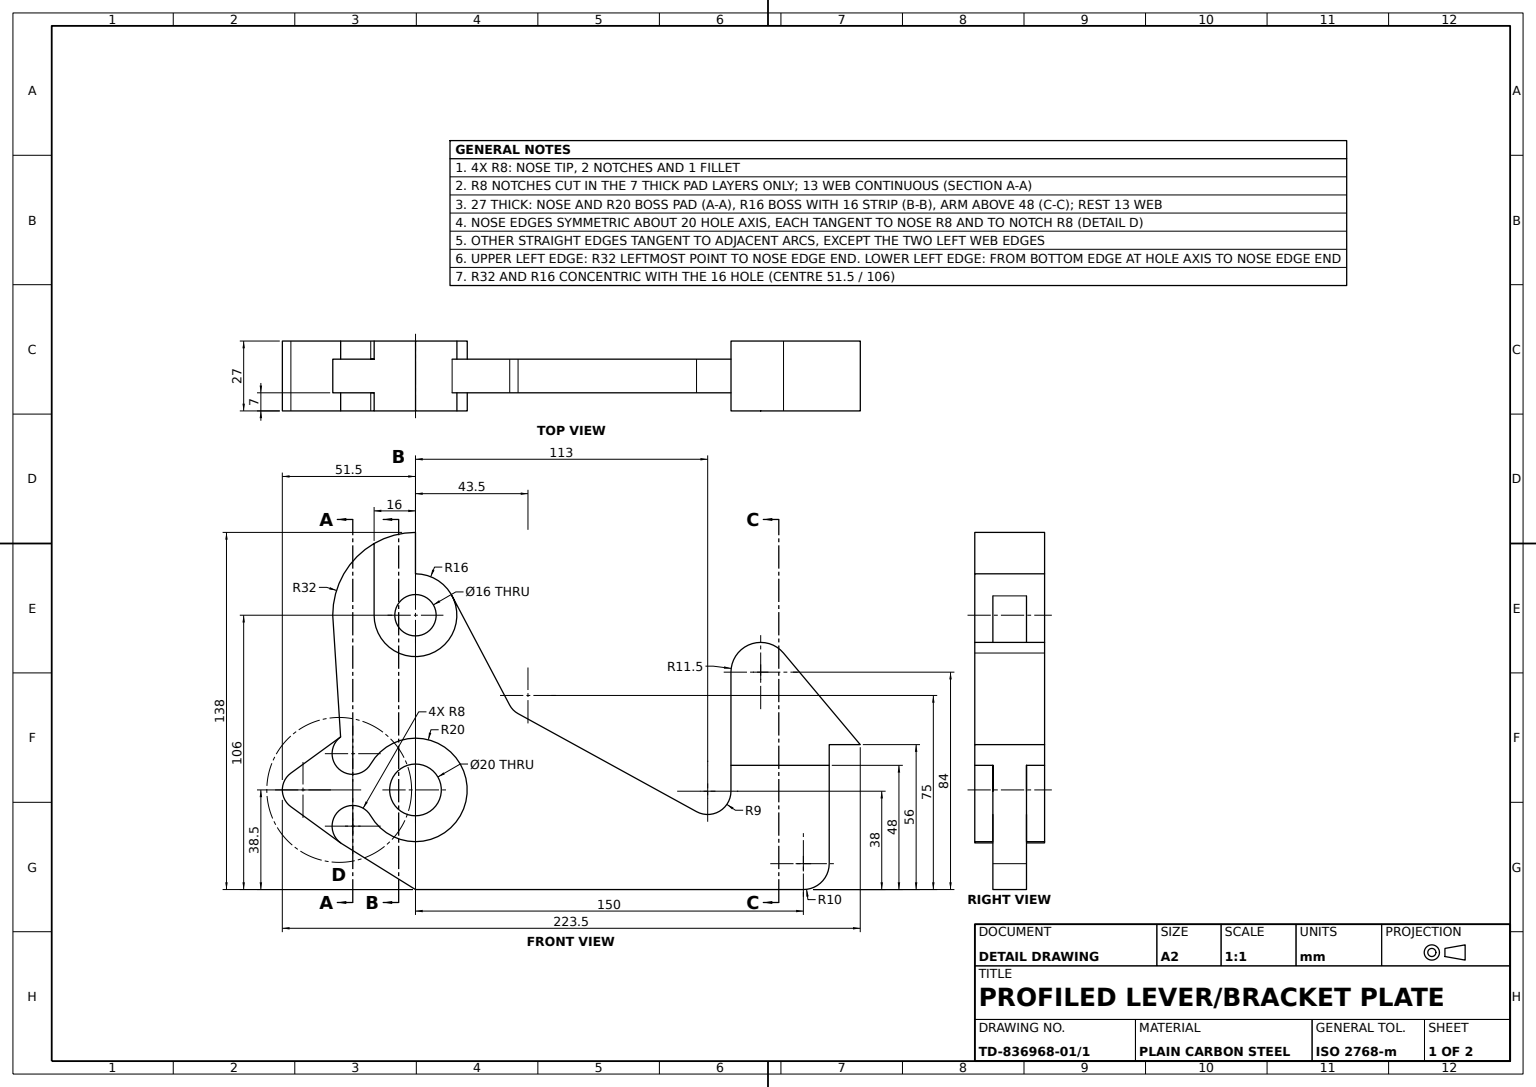
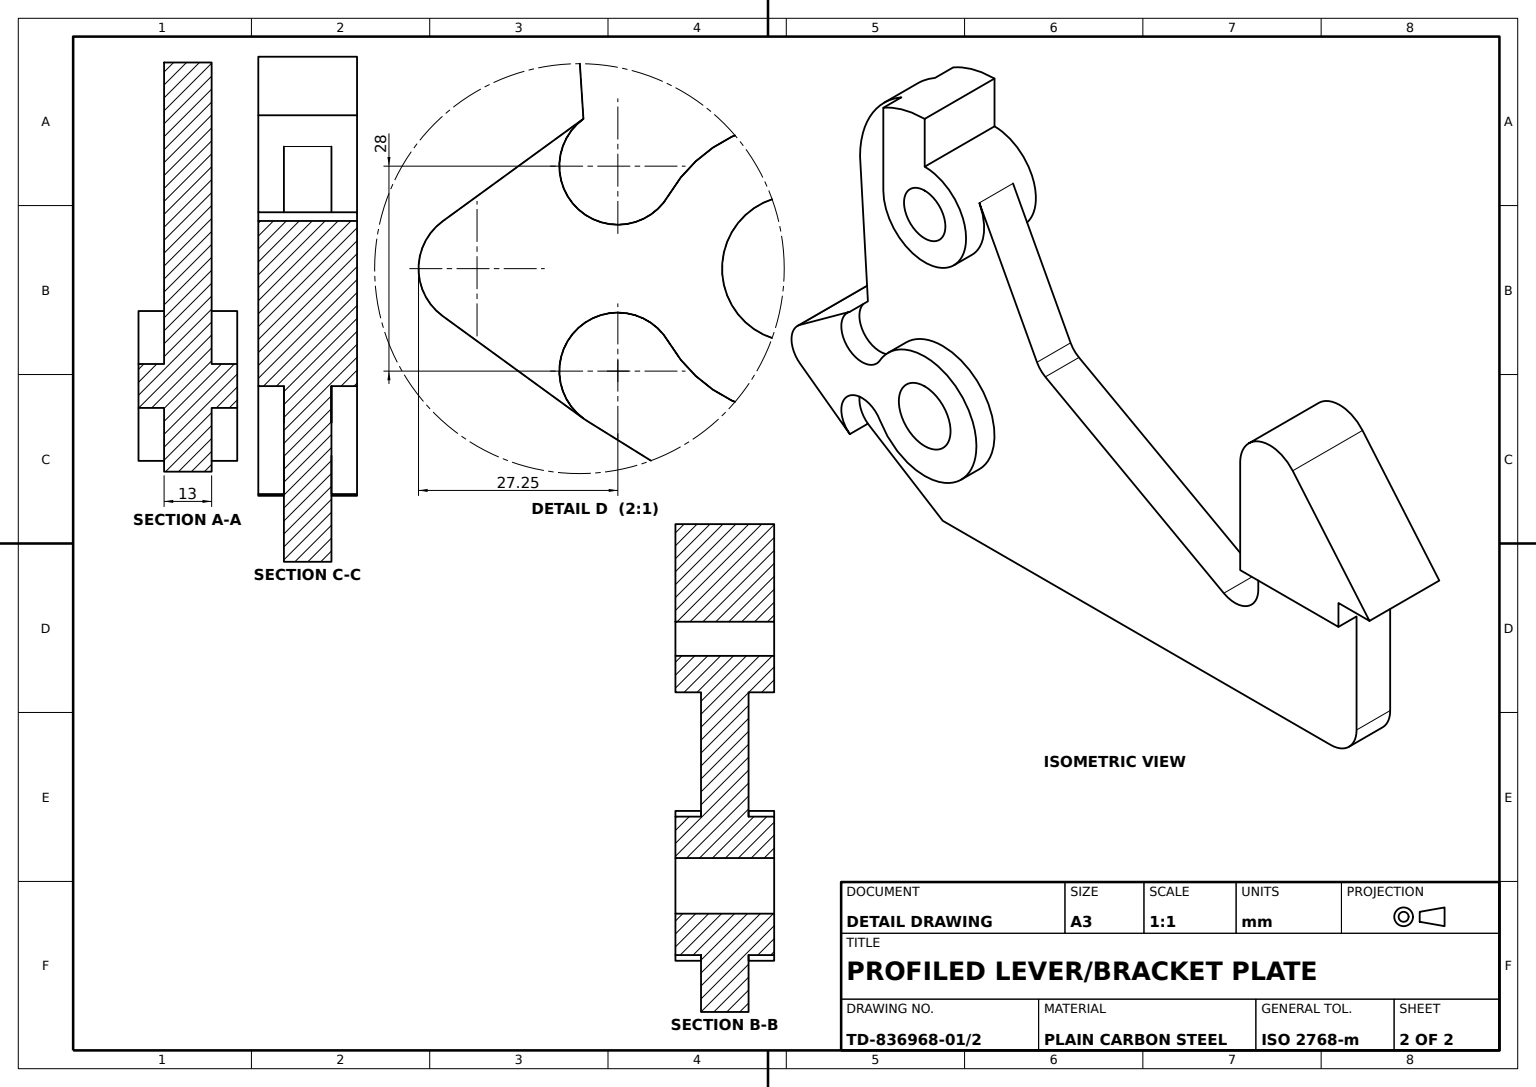
ISO-10303-21;
HEADER;
FILE_DESCRIPTION((''),'2;1');
FILE_NAME('','',(''),(''),'','','');
FILE_SCHEMA(('AUTOMOTIVE_DESIGN'));
ENDSEC;
DATA;
#1=APPLICATION_CONTEXT('');
#2=PRODUCT_CONTEXT('',#1,'mechanical');
#3=PRODUCT('','','',(#2));
#4=PRODUCT_DEFINITION_FORMATION('','',#3);
#5=PRODUCT_DEFINITION_CONTEXT('',#1,'design');
#6=PRODUCT_DEFINITION('','',#4,#5);
#7=PRODUCT_DEFINITION_SHAPE('','',#6);
#8=(LENGTH_UNIT()NAMED_UNIT(*)SI_UNIT(.MILLI.,.METRE.));
#9=(NAMED_UNIT(*)PLANE_ANGLE_UNIT()SI_UNIT($,.RADIAN.));
#10=(NAMED_UNIT(*)SI_UNIT($,.STERADIAN.)SOLID_ANGLE_UNIT());
#11=UNCERTAINTY_MEASURE_WITH_UNIT(LENGTH_MEASURE(1.E-05),#8,'distance_accuracy_value','');
#12=(GEOMETRIC_REPRESENTATION_CONTEXT(3)GLOBAL_UNCERTAINTY_ASSIGNED_CONTEXT((#11))GLOBAL_UNIT_ASSIGNED_CONTEXT((#8,#9,#10))REPRESENTATION_CONTEXT('',''));
#13=CARTESIAN_POINT('',(-178.473353,13.,-7.706444));
#14=VERTEX_POINT('',#13);
#15=CARTESIAN_POINT('',(-178.473353,0.,-7.706444));
#16=VERTEX_POINT('',#15);
#17=DIRECTION('',(0.,-1.,0.));
#18=VECTOR('',#17,1000.);
#19=LINE('',#13,#18);
#20=EDGE_CURVE('',#14,#16,#19,.T.);
#21=ORIENTED_EDGE('',*,*,#20,.T.);
#22=CARTESIAN_POINT('',(-150.,0.,10.));
#23=VERTEX_POINT('',#22);
#24=CARTESIAN_POINT('',(-46.314737,0.,74.477735));
#25=DIRECTION('',(-0.849194487,0.,-0.528080225));
#26=VECTOR('',#25,1000.);
#27=LINE('',#24,#26);
#28=EDGE_CURVE('',#23,#16,#27,.T.);
#29=ORIENTED_EDGE('',*,*,#28,.F.);
#30=CARTESIAN_POINT('',(-150.,13.,10.));
#31=VERTEX_POINT('',#30);
#32=LINE('',#30,#18);
#33=EDGE_CURVE('',#31,#23,#32,.T.);
#34=ORIENTED_EDGE('',*,*,#33,.F.);
#35=CARTESIAN_POINT('',(-46.314737,13.,74.477735));
#36=LINE('',#35,#26);
#37=EDGE_CURVE('',#31,#14,#36,.T.);
#38=ORIENTED_EDGE('',*,*,#37,.T.);
#39=EDGE_LOOP('',(#21,#29,#34,#38));
#40=FACE_OUTER_BOUND('',#39,.T.);
#41=DIRECTION('',(-0.528080225,0.,0.849194487));
#42=DIRECTION('',(0.849194487,0.,0.528080225));
#43=AXIS2_PLACEMENT_3D('',#35,#41,#42);
#44=PLANE('',#43);
#45=ADVANCED_FACE('',(#40),#44,.T.);
#46=ORIENTED_EDGE('',*,*,#37,.F.);
#47=CARTESIAN_POINT('',(0.,13.,10.));
#48=VERTEX_POINT('',#47);
#49=DIRECTION('',(-1.,0.,0.));
#50=VECTOR('',#49,1000.);
#51=LINE('',#47,#50);
#52=EDGE_CURVE('',#48,#31,#51,.T.);
#53=ORIENTED_EDGE('',*,*,#52,.F.);
#54=CARTESIAN_POINT('',(10.,13.,0.));
#55=VERTEX_POINT('',#54);
#56=CARTESIAN_POINT('',(0.,13.,0.));
#57=DIRECTION('',(0.,1.,0.));
#58=DIRECTION('',(0.,0.,1.));
#59=AXIS2_PLACEMENT_3D('',#56,#57,#58);
#60=CIRCLE('',#59,10.);
#61=EDGE_CURVE('',#48,#55,#60,.T.);
#62=ORIENTED_EDGE('',*,*,#61,.T.);
#63=CARTESIAN_POINT('',(10.,13.,-38.));
#64=VERTEX_POINT('',#63);
#65=DIRECTION('',(0.,0.,-1.));
#66=VECTOR('',#65,1000.);
#67=LINE('',#54,#66);
#68=EDGE_CURVE('',#55,#64,#67,.T.);
#69=ORIENTED_EDGE('',*,*,#68,.T.);
#70=CARTESIAN_POINT('',(-28.,13.,-38.));
#71=VERTEX_POINT('',#70);
#72=CARTESIAN_POINT('',(0.,13.,-38.));
#73=LINE('',#72,#50);
#74=EDGE_CURVE('',#64,#71,#73,.T.);
#75=ORIENTED_EDGE('',*,*,#74,.T.);
#76=CARTESIAN_POINT('',(-28.,13.,-28.));
#77=VERTEX_POINT('',#76);
#78=CARTESIAN_POINT('',(-28.,13.,0.));
#79=VECTOR('',#58,1000.);
#80=LINE('',#78,#79);
#81=EDGE_CURVE('',#71,#77,#80,.T.);
#82=ORIENTED_EDGE('',*,*,#81,.T.);
#83=CARTESIAN_POINT('',(-41.329918,13.,-20.110018));
#84=VERTEX_POINT('',#83);
#85=CARTESIAN_POINT('',(-37.,13.,-28.));
#86=AXIS2_PLACEMENT_3D('',#85,#57,#58);
#87=CIRCLE('',#86,9.);
#88=EDGE_CURVE('',#84,#77,#87,.T.);
#89=ORIENTED_EDGE('',*,*,#88,.F.);
#90=CARTESIAN_POINT('',(-110.348816,13.,-57.986683));
#91=VERTEX_POINT('',#90);
#92=CARTESIAN_POINT('',(-1.084484,13.,1.976147));
#93=DIRECTION('',(0.876664612,0.,0.481102024));
#94=VECTOR('',#93,1000.);
#95=LINE('',#92,#94);
#96=EDGE_CURVE('',#91,#84,#95,.T.);
#97=ORIENTED_EDGE('',*,*,#96,.F.);
#98=CARTESIAN_POINT('',(-113.574983,13.,-61.26575));
#99=VERTEX_POINT('',#98);
#100=CARTESIAN_POINT('',(-106.5,13.,-65.));
#101=AXIS2_PLACEMENT_3D('',#100,#57,#58);
#102=CIRCLE('',#101,8.);
#103=EDGE_CURVE('',#99,#91,#102,.T.);
#104=ORIENTED_EDGE('',*,*,#103,.F.);
#105=CARTESIAN_POINT('',(-135.850035,13.,-103.4685));
#106=VERTEX_POINT('',#105);
#107=CARTESIAN_POINT('',(-63.5377,13.,33.535862));
#108=DIRECTION('',(0.466781221,0.,0.884372824));
#109=VECTOR('',#108,1000.);
#110=LINE('',#107,#109);
#111=EDGE_CURVE('',#106,#99,#110,.T.);
#112=ORIENTED_EDGE('',*,*,#111,.F.);
#113=CARTESIAN_POINT('',(-166.,13.,-96.));
#114=VERTEX_POINT('',#113);
#115=CARTESIAN_POINT('',(-150.,13.,-96.));
#116=AXIS2_PLACEMENT_3D('',#115,#17,#58);
#117=CIRCLE('',#116,16.);
#118=EDGE_CURVE('',#106,#114,#117,.T.);
#119=ORIENTED_EDGE('',*,*,#118,.T.);
#120=CARTESIAN_POINT('',(-166.,13.,-123.712813));
#121=VERTEX_POINT('',#120);
#122=CARTESIAN_POINT('',(-166.,13.,0.));
#123=LINE('',#122,#66);
#124=EDGE_CURVE('',#114,#121,#123,.T.);
#125=ORIENTED_EDGE('',*,*,#124,.T.);
#126=CARTESIAN_POINT('',(-182.,13.,-96.));
#127=VERTEX_POINT('',#126);
#128=AXIS2_PLACEMENT_3D('',#115,#57,#58);
#129=CIRCLE('',#128,32.);
#130=EDGE_CURVE('',#121,#127,#129,.T.);
#131=ORIENTED_EDGE('',*,*,#130,.T.);
#132=CARTESIAN_POINT('',(-178.953879,13.,-48.970039));
#133=VERTEX_POINT('',#132);
#134=CARTESIAN_POINT('',(-175.047752,13.,11.337808));
#135=DIRECTION('',(0.064634366,0.,0.997909013));
#136=VECTOR('',#135,1000.);
#137=LINE('',#134,#136);
#138=EDGE_CURVE('',#127,#133,#137,.T.);
#139=ORIENTED_EDGE('',*,*,#138,.T.);
#140=CARTESIAN_POINT('',(-167.320508,13.,-38.5));
#141=VERTEX_POINT('',#140);
#142=CARTESIAN_POINT('',(-174.248711,13.,-42.5));
#143=AXIS2_PLACEMENT_3D('',#142,#57,#58);
#144=CIRCLE('',#143,8.);
#145=EDGE_CURVE('',#133,#141,#144,.T.);
#146=ORIENTED_EDGE('',*,*,#145,.T.);
#147=CARTESIAN_POINT('',(-150.,13.,-48.5));
#148=VERTEX_POINT('',#147);
#149=CARTESIAN_POINT('',(-150.,13.,-28.5));
#150=AXIS2_PLACEMENT_3D('',#149,#17,#58);
#151=CIRCLE('',#150,20.);
#152=EDGE_CURVE('',#141,#148,#151,.T.);
#153=ORIENTED_EDGE('',*,*,#152,.T.);
#154=CARTESIAN_POINT('',(-150.,13.,-8.5));
#155=VERTEX_POINT('',#154);
#156=EDGE_CURVE('',#148,#155,#151,.T.);
#157=ORIENTED_EDGE('',*,*,#156,.T.);
#158=CARTESIAN_POINT('',(-167.320508,13.,-18.5));
#159=VERTEX_POINT('',#158);
#160=EDGE_CURVE('',#155,#159,#151,.T.);
#161=ORIENTED_EDGE('',*,*,#160,.T.);
#162=CARTESIAN_POINT('',(-174.248711,13.,-22.5));
#163=VERTEX_POINT('',#162);
#164=CARTESIAN_POINT('',(-174.248711,13.,-14.5));
#165=AXIS2_PLACEMENT_3D('',#164,#57,#58);
#166=CIRCLE('',#165,8.);
#167=EDGE_CURVE('',#159,#163,#166,.T.);
#168=ORIENTED_EDGE('',*,*,#167,.T.);
#169=CARTESIAN_POINT('',(-178.953879,13.,-8.029961));
#170=VERTEX_POINT('',#169);
#171=EDGE_CURVE('',#163,#170,#166,.T.);
#172=ORIENTED_EDGE('',*,*,#171,.T.);
#173=EDGE_CURVE('',#170,#14,#166,.T.);
#174=ORIENTED_EDGE('',*,*,#173,.T.);
#175=EDGE_LOOP('',(#46,#53,#62,#69,#75,#82,#89,#97,#104,#112,#119,#125,#131,#139,#146,#153,#157,#161,#168,#172,#174));
#176=FACE_OUTER_BOUND('',#175,.T.);
#177=PLANE('',#59);
#178=ADVANCED_FACE('',(#176),#177,.T.);
#179=CARTESIAN_POINT('',(-7.689634,20.,-81.391039));
#180=VERTEX_POINT('',#179);
#181=CARTESIAN_POINT('',(-7.689634,-7.,-81.391039));
#182=VERTEX_POINT('',#181);
#183=CARTESIAN_POINT('',(-7.689634,13.,-81.391039));
#184=LINE('',#183,#18);
#185=EDGE_CURVE('',#180,#182,#184,.T.);
#186=ORIENTED_EDGE('',*,*,#185,.T.);
#187=CARTESIAN_POINT('',(-16.5,-7.,-85.5));
#188=VERTEX_POINT('',#187);
#189=CARTESIAN_POINT('',(-16.5,-7.,-74.));
#190=AXIS2_PLACEMENT_3D('',#189,#57,#65);
#191=CIRCLE('',#190,11.5);
#192=EDGE_CURVE('',#182,#188,#191,.T.);
#193=ORIENTED_EDGE('',*,*,#192,.T.);
#194=CARTESIAN_POINT('',(-16.5,20.,-85.5));
#195=VERTEX_POINT('',#194);
#196=CARTESIAN_POINT('',(-16.5,13.,-85.5));
#197=LINE('',#196,#18);
#198=EDGE_CURVE('',#195,#188,#197,.T.);
#199=ORIENTED_EDGE('',*,*,#198,.F.);
#200=CARTESIAN_POINT('',(-16.5,20.,-74.));
#201=AXIS2_PLACEMENT_3D('',#200,#57,#65);
#202=CIRCLE('',#201,11.5);
#203=EDGE_CURVE('',#180,#195,#202,.T.);
#204=ORIENTED_EDGE('',*,*,#203,.F.);
#205=EDGE_LOOP('',(#186,#193,#199,#204));
#206=FACE_OUTER_BOUND('',#205,.T.);
#207=CARTESIAN_POINT('',(-16.5,13.,-74.));
#208=AXIS2_PLACEMENT_3D('',#207,#17,#65);
#209=CYLINDRICAL_SURFACE('',#208,11.5);
#210=ADVANCED_FACE('',(#206),#209,.T.);
#211=CARTESIAN_POINT('',(-178.953879,0.,-48.970039));
#212=VERTEX_POINT('',#211);
#213=CARTESIAN_POINT('',(-167.320508,0.,-38.5));
#214=VERTEX_POINT('',#213);
#215=CARTESIAN_POINT('',(-174.248711,0.,-42.5));
#216=AXIS2_PLACEMENT_3D('',#215,#57,#58);
#217=CIRCLE('',#216,8.);
#218=EDGE_CURVE('',#212,#214,#217,.T.);
#219=ORIENTED_EDGE('',*,*,#218,.T.);
#220=CARTESIAN_POINT('',(-167.320508,-7.,-38.5));
#221=VERTEX_POINT('',#220);
#222=CARTESIAN_POINT('',(-167.320508,20.,-38.5));
#223=LINE('',#222,#18);
#224=EDGE_CURVE('',#214,#221,#223,.T.);
#225=ORIENTED_EDGE('',*,*,#224,.T.);
#226=CARTESIAN_POINT('',(-178.953879,-7.,-48.970039));
#227=VERTEX_POINT('',#226);
#228=CARTESIAN_POINT('',(-174.248711,-7.,-42.5));
#229=AXIS2_PLACEMENT_3D('',#228,#17,#58);
#230=CIRCLE('',#229,8.);
#231=EDGE_CURVE('',#221,#227,#230,.T.);
#232=ORIENTED_EDGE('',*,*,#231,.T.);
#233=CARTESIAN_POINT('',(-178.953879,20.,-48.970039));
#234=LINE('',#233,#18);
#235=EDGE_CURVE('',#212,#227,#234,.T.);
#236=ORIENTED_EDGE('',*,*,#235,.F.);
#237=EDGE_LOOP('',(#219,#225,#232,#236));
#238=FACE_OUTER_BOUND('',#237,.T.);
#239=CARTESIAN_POINT('',(-174.248711,20.,-42.5));
#240=AXIS2_PLACEMENT_3D('',#239,#17,#65);
#241=CYLINDRICAL_SURFACE('',#240,8.);
#242=ADVANCED_FACE('',(#238),#241,.F.);
#243=CARTESIAN_POINT('',(-174.248711,0.,-22.5));
#244=VERTEX_POINT('',#243);
#245=CARTESIAN_POINT('',(-174.248711,-7.,-22.5));
#246=VERTEX_POINT('',#245);
#247=CARTESIAN_POINT('',(-174.248711,20.,-22.5));
#248=LINE('',#247,#18);
#249=EDGE_CURVE('',#244,#246,#248,.T.);
#250=ORIENTED_EDGE('',*,*,#249,.T.);
#251=CARTESIAN_POINT('',(-167.320508,-7.,-18.5));
#252=VERTEX_POINT('',#251);
#253=CARTESIAN_POINT('',(-174.248711,-7.,-14.5));
#254=AXIS2_PLACEMENT_3D('',#253,#17,#58);
#255=CIRCLE('',#254,8.);
#256=EDGE_CURVE('',#246,#252,#255,.T.);
#257=ORIENTED_EDGE('',*,*,#256,.T.);
#258=CARTESIAN_POINT('',(-167.320508,0.,-18.5));
#259=VERTEX_POINT('',#258);
#260=CARTESIAN_POINT('',(-167.320508,20.,-18.5));
#261=LINE('',#260,#18);
#262=EDGE_CURVE('',#259,#252,#261,.T.);
#263=ORIENTED_EDGE('',*,*,#262,.F.);
#264=CARTESIAN_POINT('',(-174.248711,0.,-14.5));
#265=AXIS2_PLACEMENT_3D('',#264,#57,#58);
#266=CIRCLE('',#265,8.);
#267=EDGE_CURVE('',#259,#244,#266,.T.);
#268=ORIENTED_EDGE('',*,*,#267,.T.);
#269=EDGE_LOOP('',(#250,#257,#263,#268));
#270=FACE_OUTER_BOUND('',#269,.T.);
#271=CARTESIAN_POINT('',(-174.248711,20.,-14.5));
#272=AXIS2_PLACEMENT_3D('',#271,#17,#65);
#273=CYLINDRICAL_SURFACE('',#272,8.);
#274=ADVANCED_FACE('',(#270),#273,.F.);
#275=CARTESIAN_POINT('',(-150.,20.,-18.5));
#276=VERTEX_POINT('',#275);
#277=CARTESIAN_POINT('',(-150.,-7.,-18.5));
#278=VERTEX_POINT('',#277);
#279=CARTESIAN_POINT('',(-150.,13.,-18.5));
#280=LINE('',#279,#18);
#281=EDGE_CURVE('',#276,#278,#280,.T.);
#282=ORIENTED_EDGE('',*,*,#281,.T.);
#283=CARTESIAN_POINT('',(-150.,-7.,-38.5));
#284=VERTEX_POINT('',#283);
#285=CARTESIAN_POINT('',(-150.,-7.,-28.5));
#286=AXIS2_PLACEMENT_3D('',#285,#57,#58);
#287=CIRCLE('',#286,10.);
#288=EDGE_CURVE('',#284,#278,#287,.T.);
#289=ORIENTED_EDGE('',*,*,#288,.F.);
#290=CARTESIAN_POINT('',(-150.,20.,-38.5));
#291=VERTEX_POINT('',#290);
#292=CARTESIAN_POINT('',(-150.,13.,-38.5));
#293=LINE('',#292,#18);
#294=EDGE_CURVE('',#291,#284,#293,.T.);
#295=ORIENTED_EDGE('',*,*,#294,.F.);
#296=CARTESIAN_POINT('',(-150.,20.,-28.5));
#297=AXIS2_PLACEMENT_3D('',#296,#57,#58);
#298=CIRCLE('',#297,10.);
#299=EDGE_CURVE('',#291,#276,#298,.T.);
#300=ORIENTED_EDGE('',*,*,#299,.T.);
#301=EDGE_LOOP('',(#282,#289,#295,#300));
#302=FACE_OUTER_BOUND('',#301,.T.);
#303=AXIS2_PLACEMENT_3D('',#149,#17,#65);
#304=CYLINDRICAL_SURFACE('',#303,10.);
#305=ADVANCED_FACE('',(#302),#304,.F.);
#306=EDGE_CURVE('',#276,#291,#298,.T.);
#307=ORIENTED_EDGE('',*,*,#306,.T.);
#308=ORIENTED_EDGE('',*,*,#294,.T.);
#309=EDGE_CURVE('',#278,#284,#287,.T.);
#310=ORIENTED_EDGE('',*,*,#309,.F.);
#311=ORIENTED_EDGE('',*,*,#281,.F.);
#312=EDGE_LOOP('',(#307,#308,#310,#311));
#313=FACE_OUTER_BOUND('',#312,.T.);
#314=ADVANCED_FACE('',(#313),#304,.F.);
#315=CARTESIAN_POINT('',(-28.,20.,-38.));
#316=VERTEX_POINT('',#315);
#317=CARTESIAN_POINT('',(10.,20.,-38.));
#318=VERTEX_POINT('',#317);
#319=DIRECTION('',(1.,0.,0.));
#320=VECTOR('',#319,1000.);
#321=LINE('',#317,#320);
#322=EDGE_CURVE('',#316,#318,#321,.T.);
#323=ORIENTED_EDGE('',*,*,#322,.T.);
#324=CARTESIAN_POINT('',(10.,20.,-46.));
#325=VERTEX_POINT('',#324);
#326=LINE('',#324,#66);
#327=EDGE_CURVE('',#318,#325,#326,.T.);
#328=ORIENTED_EDGE('',*,*,#327,.T.);
#329=CARTESIAN_POINT('',(22.,20.,-46.));
#330=VERTEX_POINT('',#329);
#331=LINE('',#329,#320);
#332=EDGE_CURVE('',#325,#330,#331,.T.);
#333=ORIENTED_EDGE('',*,*,#332,.T.);
#334=DIRECTION('',(-0.642699021,0.,-0.766118769));
#335=VECTOR('',#334,1000.);
#336=LINE('',#179,#335);
#337=EDGE_CURVE('',#330,#180,#336,.T.);
#338=ORIENTED_EDGE('',*,*,#337,.T.);
#339=ORIENTED_EDGE('',*,*,#203,.T.);
#340=CARTESIAN_POINT('',(-28.,20.,-74.));
#341=VERTEX_POINT('',#340);
#342=EDGE_CURVE('',#195,#341,#202,.T.);
#343=ORIENTED_EDGE('',*,*,#342,.T.);
#344=LINE('',#315,#79);
#345=EDGE_CURVE('',#341,#316,#344,.T.);
#346=ORIENTED_EDGE('',*,*,#345,.T.);
#347=EDGE_LOOP('',(#323,#328,#333,#338,#339,#343,#346));
#348=FACE_OUTER_BOUND('',#347,.T.);
#349=AXIS2_PLACEMENT_3D('',#200,#17,#65);
#350=PLANE('',#349);
#351=ADVANCED_FACE('',(#348),#350,.F.);
#352=CARTESIAN_POINT('',(-198.205168,20.,-22.029961));
#353=VERTEX_POINT('',#352);
#354=CARTESIAN_POINT('',(-178.953879,20.,-8.029961));
#355=VERTEX_POINT('',#354);
#356=DIRECTION('',(0.808754813,0.,0.588145945));
#357=VECTOR('',#356,1000.);
#358=LINE('',#352,#357);
#359=EDGE_CURVE('',#353,#355,#358,.T.);
#360=ORIENTED_EDGE('',*,*,#359,.T.);
#361=VERTEX_POINT('',#247);
#362=AXIS2_PLACEMENT_3D('',#271,#17,#58);
#363=CIRCLE('',#362,8.);
#364=EDGE_CURVE('',#355,#361,#363,.T.);
#365=ORIENTED_EDGE('',*,*,#364,.T.);
#366=VERTEX_POINT('',#260);
#367=EDGE_CURVE('',#361,#366,#363,.T.);
#368=ORIENTED_EDGE('',*,*,#367,.T.);
#369=CARTESIAN_POINT('',(-150.,20.,-8.5));
#370=VERTEX_POINT('',#369);
#371=CIRCLE('',#297,20.);
#372=EDGE_CURVE('',#366,#370,#371,.T.);
#373=ORIENTED_EDGE('',*,*,#372,.T.);
#374=CARTESIAN_POINT('',(-150.,20.,-48.5));
#375=VERTEX_POINT('',#374);
#376=EDGE_CURVE('',#370,#375,#371,.T.);
#377=ORIENTED_EDGE('',*,*,#376,.T.);
#378=VERTEX_POINT('',#222);
#379=EDGE_CURVE('',#375,#378,#371,.T.);
#380=ORIENTED_EDGE('',*,*,#379,.T.);
#381=VERTEX_POINT('',#233);
#382=AXIS2_PLACEMENT_3D('',#239,#17,#58);
#383=CIRCLE('',#382,8.);
#384=EDGE_CURVE('',#378,#381,#383,.T.);
#385=ORIENTED_EDGE('',*,*,#384,.T.);
#386=CARTESIAN_POINT('',(-198.205168,20.,-34.970039));
#387=VERTEX_POINT('',#386);
#388=DIRECTION('',(-0.808754813,0.,0.588145945));
#389=VECTOR('',#388,1000.);
#390=LINE('',#386,#389);
#391=EDGE_CURVE('',#381,#387,#390,.T.);
#392=ORIENTED_EDGE('',*,*,#391,.T.);
#393=CARTESIAN_POINT('',(-193.5,20.,-28.5));
#394=AXIS2_PLACEMENT_3D('',#393,#57,#58);
#395=CIRCLE('',#394,8.);
#396=EDGE_CURVE('',#387,#353,#395,.T.);
#397=ORIENTED_EDGE('',*,*,#396,.T.);
#398=EDGE_LOOP('',(#360,#365,#368,#373,#377,#380,#385,#392,#397));
#399=FACE_OUTER_BOUND('',#398,.T.);
#400=ORIENTED_EDGE('',*,*,#306,.F.);
#401=ORIENTED_EDGE('',*,*,#299,.F.);
#402=EDGE_LOOP('',(#400,#401));
#403=FACE_BOUND('',#402,.T.);
#404=PLANE('',#394);
#405=ADVANCED_FACE('',(#399,#403),#404,.T.);
#406=CARTESIAN_POINT('',(-198.205168,-7.,-34.970039));
#407=VERTEX_POINT('',#406);
#408=CARTESIAN_POINT('',(-198.205168,13.,-34.970039));
#409=LINE('',#408,#18);
#410=EDGE_CURVE('',#387,#407,#409,.T.);
#411=ORIENTED_EDGE('',*,*,#410,.F.);
#412=ORIENTED_EDGE('',*,*,#391,.F.);
#413=EDGE_CURVE('',#381,#133,#234,.T.);
#414=ORIENTED_EDGE('',*,*,#413,.T.);
#415=LINE('',#132,#18);
#416=EDGE_CURVE('',#133,#212,#415,.T.);
#417=ORIENTED_EDGE('',*,*,#416,.T.);
#418=ORIENTED_EDGE('',*,*,#235,.T.);
#419=LINE('',#406,#389);
#420=EDGE_CURVE('',#227,#407,#419,.T.);
#421=ORIENTED_EDGE('',*,*,#420,.T.);
#422=EDGE_LOOP('',(#411,#412,#414,#417,#418,#421));
#423=FACE_OUTER_BOUND('',#422,.T.);
#424=CARTESIAN_POINT('',(-85.196323,13.,-117.152787));
#425=DIRECTION('',(-0.588145945,0.,-0.808754813));
#426=AXIS2_PLACEMENT_3D('',#424,#425,#388);
#427=PLANE('',#426);
#428=ADVANCED_FACE('',(#423),#427,.T.);
#429=LINE('',#374,#18);
#430=EDGE_CURVE('',#375,#148,#429,.T.);
#431=ORIENTED_EDGE('',*,*,#430,.F.);
#432=ORIENTED_EDGE('',*,*,#376,.F.);
#433=LINE('',#369,#18);
#434=EDGE_CURVE('',#370,#155,#433,.T.);
#435=ORIENTED_EDGE('',*,*,#434,.T.);
#436=ORIENTED_EDGE('',*,*,#156,.F.);
#437=EDGE_LOOP('',(#431,#432,#435,#436));
#438=FACE_OUTER_BOUND('',#437,.T.);
#439=AXIS2_PLACEMENT_3D('',#296,#17,#65);
#440=CYLINDRICAL_SURFACE('',#439,20.);
#441=ADVANCED_FACE('',(#438),#440,.T.);
#442=CARTESIAN_POINT('',(-178.953879,0.,-8.029961));
#443=VERTEX_POINT('',#442);
#444=LINE('',#169,#18);
#445=EDGE_CURVE('',#170,#443,#444,.T.);
#446=ORIENTED_EDGE('',*,*,#445,.T.);
#447=EDGE_CURVE('',#443,#16,#266,.T.);
#448=ORIENTED_EDGE('',*,*,#447,.T.);
#449=ORIENTED_EDGE('',*,*,#20,.F.);
#450=ORIENTED_EDGE('',*,*,#173,.F.);
#451=EDGE_LOOP('',(#446,#448,#449,#450));
#452=FACE_OUTER_BOUND('',#451,.T.);
#453=AXIS2_PLACEMENT_3D('',#164,#17,#65);
#454=CYLINDRICAL_SURFACE('',#453,8.);
#455=ADVANCED_FACE('',(#452),#454,.T.);
#456=ORIENTED_EDGE('',*,*,#52,.T.);
#457=ORIENTED_EDGE('',*,*,#33,.T.);
#458=CARTESIAN_POINT('',(0.,0.,10.));
#459=VERTEX_POINT('',#458);
#460=LINE('',#458,#50);
#461=EDGE_CURVE('',#459,#23,#460,.T.);
#462=ORIENTED_EDGE('',*,*,#461,.F.);
#463=LINE('',#47,#18);
#464=EDGE_CURVE('',#48,#459,#463,.T.);
#465=ORIENTED_EDGE('',*,*,#464,.F.);
#466=EDGE_LOOP('',(#456,#457,#462,#465));
#467=FACE_OUTER_BOUND('',#466,.T.);
#468=AXIS2_PLACEMENT_3D('',#47,#58,#319);
#469=PLANE('',#468);
#470=ADVANCED_FACE('',(#467),#469,.T.);
#471=ORIENTED_EDGE('',*,*,#138,.F.);
#472=CARTESIAN_POINT('',(-182.,0.,-96.));
#473=VERTEX_POINT('',#472);
#474=LINE('',#126,#18);
#475=EDGE_CURVE('',#127,#473,#474,.T.);
#476=ORIENTED_EDGE('',*,*,#475,.T.);
#477=CARTESIAN_POINT('',(-175.047752,0.,11.337808));
#478=LINE('',#477,#136);
#479=EDGE_CURVE('',#473,#212,#478,.T.);
#480=ORIENTED_EDGE('',*,*,#479,.T.);
#481=ORIENTED_EDGE('',*,*,#416,.F.);
#482=EDGE_LOOP('',(#471,#476,#480,#481));
#483=FACE_OUTER_BOUND('',#482,.T.);
#484=DIRECTION('',(0.997909013,0.,-0.064634366));
#485=DIRECTION('',(-0.064634366,0.,-0.997909013));
#486=AXIS2_PLACEMENT_3D('',#134,#484,#485);
#487=PLANE('',#486);
#488=ADVANCED_FACE('',(#483),#487,.F.);
#489=CARTESIAN_POINT('',(-28.,-7.,-74.));
#490=VERTEX_POINT('',#489);
#491=CARTESIAN_POINT('',(-28.,-7.,-38.));
#492=VERTEX_POINT('',#491);
#493=LINE('',#491,#79);
#494=EDGE_CURVE('',#490,#492,#493,.T.);
#495=ORIENTED_EDGE('',*,*,#494,.T.);
#496=CARTESIAN_POINT('',(-28.,0.,-38.));
#497=VERTEX_POINT('',#496);
#498=LINE('',#315,#18);
#499=EDGE_CURVE('',#497,#492,#498,.T.);
#500=ORIENTED_EDGE('',*,*,#499,.F.);
#501=CARTESIAN_POINT('',(-28.,0.,-28.));
#502=VERTEX_POINT('',#501);
#503=CARTESIAN_POINT('',(-28.,0.,0.));
#504=LINE('',#503,#79);
#505=EDGE_CURVE('',#497,#502,#504,.T.);
#506=ORIENTED_EDGE('',*,*,#505,.T.);
#507=LINE('',#76,#18);
#508=EDGE_CURVE('',#77,#502,#507,.T.);
#509=ORIENTED_EDGE('',*,*,#508,.F.);
#510=ORIENTED_EDGE('',*,*,#81,.F.);
#511=EDGE_CURVE('',#316,#71,#498,.T.);
#512=ORIENTED_EDGE('',*,*,#511,.F.);
#513=ORIENTED_EDGE('',*,*,#345,.F.);
#514=CARTESIAN_POINT('',(-28.,13.,-74.));
#515=LINE('',#514,#18);
#516=EDGE_CURVE('',#341,#490,#515,.T.);
#517=ORIENTED_EDGE('',*,*,#516,.T.);
#518=EDGE_LOOP('',(#495,#500,#506,#509,#510,#512,#513,#517));
#519=FACE_OUTER_BOUND('',#518,.T.);
#520=AXIS2_PLACEMENT_3D('',#78,#319,#65);
#521=PLANE('',#520);
#522=ADVANCED_FACE('',(#519),#521,.F.);
#523=ORIENTED_EDGE('',*,*,#516,.F.);
#524=ORIENTED_EDGE('',*,*,#342,.F.);
#525=ORIENTED_EDGE('',*,*,#198,.T.);
#526=EDGE_CURVE('',#188,#490,#191,.T.);
#527=ORIENTED_EDGE('',*,*,#526,.T.);
#528=EDGE_LOOP('',(#523,#524,#525,#527));
#529=FACE_OUTER_BOUND('',#528,.T.);
#530=ADVANCED_FACE('',(#529),#209,.T.);
#531=CARTESIAN_POINT('',(-198.205168,-7.,-22.029961));
#532=VERTEX_POINT('',#531);
#533=CARTESIAN_POINT('',(-193.5,-7.,-28.5));
#534=AXIS2_PLACEMENT_3D('',#533,#57,#58);
#535=CIRCLE('',#534,8.);
#536=EDGE_CURVE('',#407,#532,#535,.T.);
#537=ORIENTED_EDGE('',*,*,#536,.T.);
#538=CARTESIAN_POINT('',(-198.205168,13.,-22.029961));
#539=LINE('',#538,#18);
#540=EDGE_CURVE('',#353,#532,#539,.T.);
#541=ORIENTED_EDGE('',*,*,#540,.F.);
#542=ORIENTED_EDGE('',*,*,#396,.F.);
#543=ORIENTED_EDGE('',*,*,#410,.T.);
#544=EDGE_LOOP('',(#537,#541,#542,#543));
#545=FACE_OUTER_BOUND('',#544,.T.);
#546=CARTESIAN_POINT('',(-193.5,13.,-28.5));
#547=AXIS2_PLACEMENT_3D('',#546,#17,#65);
#548=CYLINDRICAL_SURFACE('',#547,8.);
#549=ADVANCED_FACE('',(#545),#548,.T.);
#550=CARTESIAN_POINT('',(10.,-7.,-38.));
#551=VERTEX_POINT('',#550);
#552=LINE('',#550,#320);
#553=EDGE_CURVE('',#492,#551,#552,.T.);
#554=ORIENTED_EDGE('',*,*,#553,.F.);
#555=ORIENTED_EDGE('',*,*,#494,.F.);
#556=ORIENTED_EDGE('',*,*,#526,.F.);
#557=ORIENTED_EDGE('',*,*,#192,.F.);
#558=CARTESIAN_POINT('',(22.,-7.,-46.));
#559=VERTEX_POINT('',#558);
#560=LINE('',#181,#335);
#561=EDGE_CURVE('',#559,#182,#560,.T.);
#562=ORIENTED_EDGE('',*,*,#561,.F.);
#563=CARTESIAN_POINT('',(10.,-7.,-46.));
#564=VERTEX_POINT('',#563);
#565=LINE('',#558,#320);
#566=EDGE_CURVE('',#564,#559,#565,.T.);
#567=ORIENTED_EDGE('',*,*,#566,.F.);
#568=LINE('',#563,#66);
#569=EDGE_CURVE('',#551,#564,#568,.T.);
#570=ORIENTED_EDGE('',*,*,#569,.F.);
#571=EDGE_LOOP('',(#554,#555,#556,#557,#562,#567,#570));
#572=FACE_OUTER_BOUND('',#571,.T.);
#573=AXIS2_PLACEMENT_3D('',#189,#17,#65);
#574=PLANE('',#573);
#575=ADVANCED_FACE('',(#572),#574,.T.);
#576=ORIENTED_EDGE('',*,*,#327,.F.);
#577=LINE('',#317,#18);
#578=EDGE_CURVE('',#318,#64,#577,.T.);
#579=ORIENTED_EDGE('',*,*,#578,.T.);
#580=ORIENTED_EDGE('',*,*,#68,.F.);
#581=CARTESIAN_POINT('',(10.,0.,0.));
#582=VERTEX_POINT('',#581);
#583=LINE('',#54,#18);
#584=EDGE_CURVE('',#55,#582,#583,.T.);
#585=ORIENTED_EDGE('',*,*,#584,.T.);
#586=CARTESIAN_POINT('',(10.,0.,-38.));
#587=VERTEX_POINT('',#586);
#588=LINE('',#581,#66);
#589=EDGE_CURVE('',#582,#587,#588,.T.);
#590=ORIENTED_EDGE('',*,*,#589,.T.);
#591=EDGE_CURVE('',#587,#551,#577,.T.);
#592=ORIENTED_EDGE('',*,*,#591,.T.);
#593=ORIENTED_EDGE('',*,*,#569,.T.);
#594=CARTESIAN_POINT('',(10.,13.,-46.));
#595=LINE('',#594,#18);
#596=EDGE_CURVE('',#325,#564,#595,.T.);
#597=ORIENTED_EDGE('',*,*,#596,.F.);
#598=EDGE_LOOP('',(#576,#579,#580,#585,#590,#592,#593,#597));
#599=FACE_OUTER_BOUND('',#598,.T.);
#600=AXIS2_PLACEMENT_3D('',#54,#49,#58);
#601=PLANE('',#600);
#602=ADVANCED_FACE('',(#599),#601,.F.);
#603=CARTESIAN_POINT('',(-150.,0.,-8.5));
#604=VERTEX_POINT('',#603);
#605=CARTESIAN_POINT('',(-150.,-7.,-8.5));
#606=VERTEX_POINT('',#605);
#607=EDGE_CURVE('',#604,#606,#433,.T.);
#608=ORIENTED_EDGE('',*,*,#607,.T.);
#609=CARTESIAN_POINT('',(-150.,-7.,-48.5));
#610=VERTEX_POINT('',#609);
#611=CIRCLE('',#286,20.);
#612=EDGE_CURVE('',#606,#610,#611,.T.);
#613=ORIENTED_EDGE('',*,*,#612,.T.);
#614=CARTESIAN_POINT('',(-150.,0.,-48.5));
#615=VERTEX_POINT('',#614);
#616=EDGE_CURVE('',#615,#610,#429,.T.);
#617=ORIENTED_EDGE('',*,*,#616,.F.);
#618=CARTESIAN_POINT('',(-150.,0.,-28.5));
#619=AXIS2_PLACEMENT_3D('',#618,#17,#58);
#620=CIRCLE('',#619,20.);
#621=EDGE_CURVE('',#615,#604,#620,.T.);
#622=ORIENTED_EDGE('',*,*,#621,.T.);
#623=EDGE_LOOP('',(#608,#613,#617,#622));
#624=FACE_OUTER_BOUND('',#623,.T.);
#625=ADVANCED_FACE('',(#624),#440,.T.);
#626=CARTESIAN_POINT('',(-110.348816,0.,-57.986683));
#627=VERTEX_POINT('',#626);
#628=CARTESIAN_POINT('',(-41.329918,0.,-20.110018));
#629=VERTEX_POINT('',#628);
#630=CARTESIAN_POINT('',(-1.084484,0.,1.976147));
#631=LINE('',#630,#94);
#632=EDGE_CURVE('',#627,#629,#631,.T.);
#633=ORIENTED_EDGE('',*,*,#632,.F.);
#634=LINE('',#90,#18);
#635=EDGE_CURVE('',#91,#627,#634,.T.);
#636=ORIENTED_EDGE('',*,*,#635,.F.);
#637=ORIENTED_EDGE('',*,*,#96,.T.);
#638=LINE('',#83,#18);
#639=EDGE_CURVE('',#84,#629,#638,.T.);
#640=ORIENTED_EDGE('',*,*,#639,.T.);
#641=EDGE_LOOP('',(#633,#636,#637,#640));
#642=FACE_OUTER_BOUND('',#641,.T.);
#643=DIRECTION('',(0.481102024,0.,-0.876664612));
#644=DIRECTION('',(-0.876664612,0.,-0.481102024));
#645=AXIS2_PLACEMENT_3D('',#92,#643,#644);
#646=PLANE('',#645);
#647=ADVANCED_FACE('',(#642),#646,.T.);
#648=CARTESIAN_POINT('',(-166.,20.,-96.));
#649=VERTEX_POINT('',#648);
#650=CARTESIAN_POINT('',(-150.,20.,-112.));
#651=VERTEX_POINT('',#650);
#652=CARTESIAN_POINT('',(-150.,20.,-96.));
#653=AXIS2_PLACEMENT_3D('',#652,#57,#58);
#654=CIRCLE('',#653,16.);
#655=EDGE_CURVE('',#649,#651,#654,.T.);
#656=ORIENTED_EDGE('',*,*,#655,.F.);
#657=LINE('',#648,#18);
#658=EDGE_CURVE('',#649,#114,#657,.T.);
#659=ORIENTED_EDGE('',*,*,#658,.T.);
#660=ORIENTED_EDGE('',*,*,#118,.F.);
#661=CARTESIAN_POINT('',(-135.850035,0.,-103.4685));
#662=VERTEX_POINT('',#661);
#663=LINE('',#105,#18);
#664=EDGE_CURVE('',#106,#662,#663,.T.);
#665=ORIENTED_EDGE('',*,*,#664,.T.);
#666=CARTESIAN_POINT('',(-166.,0.,-96.));
#667=VERTEX_POINT('',#666);
#668=CARTESIAN_POINT('',(-150.,0.,-96.));
#669=AXIS2_PLACEMENT_3D('',#668,#17,#58);
#670=CIRCLE('',#669,16.);
#671=EDGE_CURVE('',#662,#667,#670,.T.);
#672=ORIENTED_EDGE('',*,*,#671,.T.);
#673=CARTESIAN_POINT('',(-166.,-7.,-96.));
#674=VERTEX_POINT('',#673);
#675=EDGE_CURVE('',#667,#674,#657,.T.);
#676=ORIENTED_EDGE('',*,*,#675,.T.);
#677=CARTESIAN_POINT('',(-150.,-7.,-112.));
#678=VERTEX_POINT('',#677);
#679=CARTESIAN_POINT('',(-150.,-7.,-96.));
#680=AXIS2_PLACEMENT_3D('',#679,#57,#58);
#681=CIRCLE('',#680,16.);
#682=EDGE_CURVE('',#674,#678,#681,.T.);
#683=ORIENTED_EDGE('',*,*,#682,.T.);
#684=CARTESIAN_POINT('',(-150.,13.,-112.));
#685=LINE('',#684,#18);
#686=EDGE_CURVE('',#651,#678,#685,.T.);
#687=ORIENTED_EDGE('',*,*,#686,.F.);
#688=EDGE_LOOP('',(#656,#659,#660,#665,#672,#676,#683,#687));
#689=FACE_OUTER_BOUND('',#688,.T.);
#690=AXIS2_PLACEMENT_3D('',#115,#17,#65);
#691=CYLINDRICAL_SURFACE('',#690,16.);
#692=ADVANCED_FACE('',(#689),#691,.T.);
#693=ORIENTED_EDGE('',*,*,#616,.T.);
#694=EDGE_CURVE('',#610,#221,#611,.T.);
#695=ORIENTED_EDGE('',*,*,#694,.T.);
#696=ORIENTED_EDGE('',*,*,#224,.F.);
#697=EDGE_CURVE('',#214,#615,#620,.T.);
#698=ORIENTED_EDGE('',*,*,#697,.T.);
#699=EDGE_LOOP('',(#693,#695,#696,#698));
#700=FACE_OUTER_BOUND('',#699,.T.);
#701=ADVANCED_FACE('',(#700),#440,.T.);
#702=ORIENTED_EDGE('',*,*,#578,.F.);
#703=ORIENTED_EDGE('',*,*,#322,.F.);
#704=ORIENTED_EDGE('',*,*,#511,.T.);
#705=ORIENTED_EDGE('',*,*,#74,.F.);
#706=EDGE_LOOP('',(#702,#703,#704,#705));
#707=FACE_OUTER_BOUND('',#706,.T.);
#708=AXIS2_PLACEMENT_3D('',#317,#65,#49);
#709=PLANE('',#708);
#710=ADVANCED_FACE('',(#707),#709,.F.);
#711=ORIENTED_EDGE('',*,*,#152,.F.);
#712=EDGE_CURVE('',#378,#141,#223,.T.);
#713=ORIENTED_EDGE('',*,*,#712,.F.);
#714=ORIENTED_EDGE('',*,*,#379,.F.);
#715=ORIENTED_EDGE('',*,*,#430,.T.);
#716=EDGE_LOOP('',(#711,#713,#714,#715));
#717=FACE_OUTER_BOUND('',#716,.T.);
#718=ADVANCED_FACE('',(#717),#440,.T.);
#719=ORIENTED_EDGE('',*,*,#499,.T.);
#720=ORIENTED_EDGE('',*,*,#553,.T.);
#721=ORIENTED_EDGE('',*,*,#591,.F.);
#722=CARTESIAN_POINT('',(0.,0.,-38.));
#723=LINE('',#722,#50);
#724=EDGE_CURVE('',#587,#497,#723,.T.);
#725=ORIENTED_EDGE('',*,*,#724,.T.);
#726=EDGE_LOOP('',(#719,#720,#721,#725));
#727=FACE_OUTER_BOUND('',#726,.T.);
#728=ADVANCED_FACE('',(#727),#709,.F.);
#729=EDGE_CURVE('',#244,#443,#266,.T.);
#730=ORIENTED_EDGE('',*,*,#729,.T.);
#731=CARTESIAN_POINT('',(-178.953879,-7.,-8.029961));
#732=VERTEX_POINT('',#731);
#733=LINE('',#354,#18);
#734=EDGE_CURVE('',#443,#732,#733,.T.);
#735=ORIENTED_EDGE('',*,*,#734,.T.);
#736=EDGE_CURVE('',#732,#246,#255,.T.);
#737=ORIENTED_EDGE('',*,*,#736,.T.);
#738=ORIENTED_EDGE('',*,*,#249,.F.);
#739=EDGE_LOOP('',(#730,#735,#737,#738));
#740=FACE_OUTER_BOUND('',#739,.T.);
#741=ADVANCED_FACE('',(#740),#273,.F.);
#742=ORIENTED_EDGE('',*,*,#167,.F.);
#743=EDGE_CURVE('',#366,#159,#261,.T.);
#744=ORIENTED_EDGE('',*,*,#743,.F.);
#745=ORIENTED_EDGE('',*,*,#367,.F.);
#746=EDGE_CURVE('',#361,#163,#248,.T.);
#747=ORIENTED_EDGE('',*,*,#746,.T.);
#748=EDGE_LOOP('',(#742,#744,#745,#747));
#749=FACE_OUTER_BOUND('',#748,.T.);
#750=ADVANCED_FACE('',(#749),#273,.F.);
#751=CARTESIAN_POINT('',(-166.,20.,-123.712813));
#752=VERTEX_POINT('',#751);
#753=LINE('',#648,#79);
#754=EDGE_CURVE('',#752,#649,#753,.T.);
#755=ORIENTED_EDGE('',*,*,#754,.F.);
#756=LINE('',#751,#18);
#757=EDGE_CURVE('',#752,#121,#756,.T.);
#758=ORIENTED_EDGE('',*,*,#757,.T.);
#759=ORIENTED_EDGE('',*,*,#124,.F.);
#760=ORIENTED_EDGE('',*,*,#658,.F.);
#761=EDGE_LOOP('',(#755,#758,#759,#760));
#762=FACE_OUTER_BOUND('',#761,.T.);
#763=AXIS2_PLACEMENT_3D('',#648,#319,#65);
#764=PLANE('',#763);
#765=ADVANCED_FACE('',(#762),#764,.F.);
#766=CARTESIAN_POINT('',(22.,13.,-46.));
#767=LINE('',#766,#18);
#768=EDGE_CURVE('',#330,#559,#767,.T.);
#769=ORIENTED_EDGE('',*,*,#768,.F.);
#770=ORIENTED_EDGE('',*,*,#332,.F.);
#771=ORIENTED_EDGE('',*,*,#596,.T.);
#772=ORIENTED_EDGE('',*,*,#566,.T.);
#773=EDGE_LOOP('',(#769,#770,#771,#772));
#774=FACE_OUTER_BOUND('',#773,.T.);
#775=CARTESIAN_POINT('',(0.,13.,-46.));
#776=AXIS2_PLACEMENT_3D('',#775,#65,#49);
#777=PLANE('',#776);
#778=ADVANCED_FACE('',(#774),#777,.F.);
#779=ORIENTED_EDGE('',*,*,#171,.F.);
#780=ORIENTED_EDGE('',*,*,#746,.F.);
#781=ORIENTED_EDGE('',*,*,#364,.F.);
#782=EDGE_CURVE('',#355,#170,#733,.T.);
#783=ORIENTED_EDGE('',*,*,#782,.T.);
#784=EDGE_LOOP('',(#779,#780,#781,#783));
#785=FACE_OUTER_BOUND('',#784,.T.);
#786=ADVANCED_FACE('',(#785),#273,.F.);
#787=ORIENTED_EDGE('',*,*,#103,.T.);
#788=ORIENTED_EDGE('',*,*,#635,.T.);
#789=CARTESIAN_POINT('',(-113.574983,0.,-61.26575));
#790=VERTEX_POINT('',#789);
#791=CARTESIAN_POINT('',(-106.5,0.,-65.));
#792=AXIS2_PLACEMENT_3D('',#791,#57,#58);
#793=CIRCLE('',#792,8.);
#794=EDGE_CURVE('',#790,#627,#793,.T.);
#795=ORIENTED_EDGE('',*,*,#794,.F.);
#796=LINE('',#98,#18);
#797=EDGE_CURVE('',#99,#790,#796,.T.);
#798=ORIENTED_EDGE('',*,*,#797,.F.);
#799=EDGE_LOOP('',(#787,#788,#795,#798));
#800=FACE_OUTER_BOUND('',#799,.T.);
#801=AXIS2_PLACEMENT_3D('',#100,#17,#65);
#802=CYLINDRICAL_SURFACE('',#801,8.);
#803=ADVANCED_FACE('',(#800),#802,.F.);
#804=CARTESIAN_POINT('',(-150.,-7.,-88.));
#805=VERTEX_POINT('',#804);
#806=CARTESIAN_POINT('',(-150.,-7.,-104.));
#807=VERTEX_POINT('',#806);
#808=CIRCLE('',#680,8.);
#809=EDGE_CURVE('',#805,#807,#808,.T.);
#810=ORIENTED_EDGE('',*,*,#809,.F.);
#811=CARTESIAN_POINT('',(-150.,20.,-88.));
#812=VERTEX_POINT('',#811);
#813=CARTESIAN_POINT('',(-150.,13.,-88.));
#814=LINE('',#813,#18);
#815=EDGE_CURVE('',#812,#805,#814,.T.);
#816=ORIENTED_EDGE('',*,*,#815,.F.);
#817=CARTESIAN_POINT('',(-150.,20.,-104.));
#818=VERTEX_POINT('',#817);
#819=CIRCLE('',#653,8.);
#820=EDGE_CURVE('',#812,#818,#819,.T.);
#821=ORIENTED_EDGE('',*,*,#820,.T.);
#822=CARTESIAN_POINT('',(-150.,13.,-104.));
#823=LINE('',#822,#18);
#824=EDGE_CURVE('',#818,#807,#823,.T.);
#825=ORIENTED_EDGE('',*,*,#824,.T.);
#826=EDGE_LOOP('',(#810,#816,#821,#825));
#827=FACE_OUTER_BOUND('',#826,.T.);
#828=CYLINDRICAL_SURFACE('',#690,8.);
#829=ADVANCED_FACE('',(#827),#828,.F.);
#830=EDGE_CURVE('',#807,#805,#808,.T.);
#831=ORIENTED_EDGE('',*,*,#830,.T.);
#832=ORIENTED_EDGE('',*,*,#809,.T.);
#833=EDGE_LOOP('',(#831,#832));
#834=FACE_BOUND('',#833,.T.);
#835=ORIENTED_EDGE('',*,*,#682,.F.);
#836=CARTESIAN_POINT('',(-166.,-7.,-123.712813));
#837=VERTEX_POINT('',#836);
#838=LINE('',#673,#79);
#839=EDGE_CURVE('',#837,#674,#838,.T.);
#840=ORIENTED_EDGE('',*,*,#839,.F.);
#841=CARTESIAN_POINT('',(-150.,-7.,-128.));
#842=VERTEX_POINT('',#841);
#843=CIRCLE('',#680,32.);
#844=EDGE_CURVE('',#842,#837,#843,.T.);
#845=ORIENTED_EDGE('',*,*,#844,.F.);
#846=LINE('',#677,#66);
#847=EDGE_CURVE('',#678,#842,#846,.T.);
#848=ORIENTED_EDGE('',*,*,#847,.F.);
#849=EDGE_LOOP('',(#835,#840,#845,#848));
#850=FACE_OUTER_BOUND('',#849,.T.);
#851=PLANE('',#680);
#852=ADVANCED_FACE('',(#834,#850),#851,.F.);
#853=ORIENTED_EDGE('',*,*,#743,.T.);
#854=ORIENTED_EDGE('',*,*,#160,.F.);
#855=ORIENTED_EDGE('',*,*,#434,.F.);
#856=ORIENTED_EDGE('',*,*,#372,.F.);
#857=EDGE_LOOP('',(#853,#854,#855,#856));
#858=FACE_OUTER_BOUND('',#857,.T.);
#859=ADVANCED_FACE('',(#858),#440,.T.);
#860=ORIENTED_EDGE('',*,*,#824,.F.);
#861=EDGE_CURVE('',#818,#812,#819,.T.);
#862=ORIENTED_EDGE('',*,*,#861,.T.);
#863=ORIENTED_EDGE('',*,*,#815,.T.);
#864=ORIENTED_EDGE('',*,*,#830,.F.);
#865=EDGE_LOOP('',(#860,#862,#863,#864));
#866=FACE_OUTER_BOUND('',#865,.T.);
#867=ADVANCED_FACE('',(#866),#828,.F.);
#868=CARTESIAN_POINT('',(-166.,0.,-123.712813));
#869=VERTEX_POINT('',#868);
#870=CARTESIAN_POINT('',(-166.,0.,0.));
#871=LINE('',#870,#66);
#872=EDGE_CURVE('',#667,#869,#871,.T.);
#873=ORIENTED_EDGE('',*,*,#872,.F.);
#874=ORIENTED_EDGE('',*,*,#671,.F.);
#875=CARTESIAN_POINT('',(-63.5377,0.,33.535862));
#876=LINE('',#875,#109);
#877=EDGE_CURVE('',#662,#790,#876,.T.);
#878=ORIENTED_EDGE('',*,*,#877,.T.);
#879=ORIENTED_EDGE('',*,*,#794,.T.);
#880=ORIENTED_EDGE('',*,*,#632,.T.);
#881=CARTESIAN_POINT('',(-37.,0.,-28.));
#882=AXIS2_PLACEMENT_3D('',#881,#57,#58);
#883=CIRCLE('',#882,9.);
#884=EDGE_CURVE('',#629,#502,#883,.T.);
#885=ORIENTED_EDGE('',*,*,#884,.T.);
#886=ORIENTED_EDGE('',*,*,#505,.F.);
#887=ORIENTED_EDGE('',*,*,#724,.F.);
#888=ORIENTED_EDGE('',*,*,#589,.F.);
#889=CARTESIAN_POINT('',(0.,0.,0.));
#890=AXIS2_PLACEMENT_3D('',#889,#57,#58);
#891=CIRCLE('',#890,10.);
#892=EDGE_CURVE('',#459,#582,#891,.T.);
#893=ORIENTED_EDGE('',*,*,#892,.F.);
#894=ORIENTED_EDGE('',*,*,#461,.T.);
#895=ORIENTED_EDGE('',*,*,#28,.T.);
#896=ORIENTED_EDGE('',*,*,#447,.F.);
#897=ORIENTED_EDGE('',*,*,#729,.F.);
#898=ORIENTED_EDGE('',*,*,#267,.F.);
#899=EDGE_CURVE('',#604,#259,#620,.T.);
#900=ORIENTED_EDGE('',*,*,#899,.F.);
#901=ORIENTED_EDGE('',*,*,#621,.F.);
#902=ORIENTED_EDGE('',*,*,#697,.F.);
#903=ORIENTED_EDGE('',*,*,#218,.F.);
#904=ORIENTED_EDGE('',*,*,#479,.F.);
#905=AXIS2_PLACEMENT_3D('',#668,#57,#58);
#906=CIRCLE('',#905,32.);
#907=EDGE_CURVE('',#869,#473,#906,.T.);
#908=ORIENTED_EDGE('',*,*,#907,.F.);
#909=EDGE_LOOP('',(#873,#874,#878,#879,#880,#885,#886,#887,#888,#893,#894,#895,#896,#897,#898,#900,#901,#902,#903,#904,#908));
#910=FACE_OUTER_BOUND('',#909,.T.);
#911=PLANE('',#890);
#912=ADVANCED_FACE('',(#910),#911,.F.);
#913=CARTESIAN_POINT('',(-150.,20.,-128.));
#914=VERTEX_POINT('',#913);
#915=LINE('',#650,#66);
#916=EDGE_CURVE('',#651,#914,#915,.T.);
#917=ORIENTED_EDGE('',*,*,#916,.F.);
#918=ORIENTED_EDGE('',*,*,#686,.T.);
#919=ORIENTED_EDGE('',*,*,#847,.T.);
#920=CARTESIAN_POINT('',(-150.,13.,-128.));
#921=LINE('',#920,#18);
#922=EDGE_CURVE('',#914,#842,#921,.T.);
#923=ORIENTED_EDGE('',*,*,#922,.F.);
#924=EDGE_LOOP('',(#917,#918,#919,#923));
#925=FACE_OUTER_BOUND('',#924,.T.);
#926=CARTESIAN_POINT('',(-150.,13.,0.));
#927=AXIS2_PLACEMENT_3D('',#926,#49,#58);
#928=PLANE('',#927);
#929=ADVANCED_FACE('',(#925),#928,.F.);
#930=ORIENTED_EDGE('',*,*,#782,.F.);
#931=ORIENTED_EDGE('',*,*,#359,.F.);
#932=ORIENTED_EDGE('',*,*,#540,.T.);
#933=LINE('',#531,#357);
#934=EDGE_CURVE('',#532,#732,#933,.T.);
#935=ORIENTED_EDGE('',*,*,#934,.T.);
#936=ORIENTED_EDGE('',*,*,#734,.F.);
#937=ORIENTED_EDGE('',*,*,#445,.F.);
#938=EDGE_LOOP('',(#930,#931,#932,#935,#936,#937));
#939=FACE_OUTER_BOUND('',#938,.T.);
#940=CARTESIAN_POINT('',(-58.083369,13.,79.869979));
#941=DIRECTION('',(0.588145945,0.,-0.808754813));
#942=DIRECTION('',(-0.808754813,0.,-0.588145945));
#943=AXIS2_PLACEMENT_3D('',#940,#941,#942);
#944=PLANE('',#943);
#945=ADVANCED_FACE('',(#939),#944,.F.);
#946=ORIENTED_EDGE('',*,*,#712,.T.);
#947=ORIENTED_EDGE('',*,*,#145,.F.);
#948=ORIENTED_EDGE('',*,*,#413,.F.);
#949=ORIENTED_EDGE('',*,*,#384,.F.);
#950=EDGE_LOOP('',(#946,#947,#948,#949));
#951=FACE_OUTER_BOUND('',#950,.T.);
#952=ADVANCED_FACE('',(#951),#241,.F.);
#953=ORIENTED_EDGE('',*,*,#861,.F.);
#954=ORIENTED_EDGE('',*,*,#820,.F.);
#955=EDGE_LOOP('',(#953,#954));
#956=FACE_BOUND('',#955,.T.);
#957=ORIENTED_EDGE('',*,*,#655,.T.);
#958=ORIENTED_EDGE('',*,*,#916,.T.);
#959=CIRCLE('',#653,32.);
#960=EDGE_CURVE('',#914,#752,#959,.T.);
#961=ORIENTED_EDGE('',*,*,#960,.T.);
#962=ORIENTED_EDGE('',*,*,#754,.T.);
#963=EDGE_LOOP('',(#957,#958,#961,#962));
#964=FACE_OUTER_BOUND('',#963,.T.);
#965=PLANE('',#653);
#966=ADVANCED_FACE('',(#956,#964),#965,.T.);
#967=ORIENTED_EDGE('',*,*,#899,.T.);
#968=ORIENTED_EDGE('',*,*,#262,.T.);
#969=EDGE_CURVE('',#252,#606,#611,.T.);
#970=ORIENTED_EDGE('',*,*,#969,.T.);
#971=ORIENTED_EDGE('',*,*,#607,.F.);
#972=EDGE_LOOP('',(#967,#968,#970,#971));
#973=FACE_OUTER_BOUND('',#972,.T.);
#974=ADVANCED_FACE('',(#973),#440,.T.);
#975=ORIENTED_EDGE('',*,*,#797,.T.);
#976=ORIENTED_EDGE('',*,*,#877,.F.);
#977=ORIENTED_EDGE('',*,*,#664,.F.);
#978=ORIENTED_EDGE('',*,*,#111,.T.);
#979=EDGE_LOOP('',(#975,#976,#977,#978));
#980=FACE_OUTER_BOUND('',#979,.T.);
#981=DIRECTION('',(0.884372824,0.,-0.466781221));
#982=DIRECTION('',(-0.466781221,0.,-0.884372824));
#983=AXIS2_PLACEMENT_3D('',#107,#981,#982);
#984=PLANE('',#983);
#985=ADVANCED_FACE('',(#980),#984,.T.);
#986=ORIENTED_EDGE('',*,*,#675,.F.);
#987=ORIENTED_EDGE('',*,*,#872,.T.);
#988=EDGE_CURVE('',#869,#837,#756,.T.);
#989=ORIENTED_EDGE('',*,*,#988,.T.);
#990=ORIENTED_EDGE('',*,*,#839,.T.);
#991=EDGE_LOOP('',(#986,#987,#989,#990));
#992=FACE_OUTER_BOUND('',#991,.T.);
#993=ADVANCED_FACE('',(#992),#764,.F.);
#994=ORIENTED_EDGE('',*,*,#475,.F.);
#995=ORIENTED_EDGE('',*,*,#130,.F.);
#996=ORIENTED_EDGE('',*,*,#757,.F.);
#997=ORIENTED_EDGE('',*,*,#960,.F.);
#998=ORIENTED_EDGE('',*,*,#922,.T.);
#999=ORIENTED_EDGE('',*,*,#844,.T.);
#1000=ORIENTED_EDGE('',*,*,#988,.F.);
#1001=ORIENTED_EDGE('',*,*,#907,.T.);
#1002=EDGE_LOOP('',(#994,#995,#996,#997,#998,#999,#1000,#1001));
#1003=FACE_OUTER_BOUND('',#1002,.T.);
#1004=CYLINDRICAL_SURFACE('',#690,32.);
#1005=ADVANCED_FACE('',(#1003),#1004,.T.);
#1006=ORIENTED_EDGE('',*,*,#464,.T.);
#1007=ORIENTED_EDGE('',*,*,#892,.T.);
#1008=ORIENTED_EDGE('',*,*,#584,.F.);
#1009=ORIENTED_EDGE('',*,*,#61,.F.);
#1010=EDGE_LOOP('',(#1006,#1007,#1008,#1009));
#1011=FACE_OUTER_BOUND('',#1010,.T.);
#1012=AXIS2_PLACEMENT_3D('',#56,#17,#65);
#1013=CYLINDRICAL_SURFACE('',#1012,10.);
#1014=ADVANCED_FACE('',(#1011),#1013,.T.);
#1015=ORIENTED_EDGE('',*,*,#736,.F.);
#1016=ORIENTED_EDGE('',*,*,#934,.F.);
#1017=ORIENTED_EDGE('',*,*,#536,.F.);
#1018=ORIENTED_EDGE('',*,*,#420,.F.);
#1019=ORIENTED_EDGE('',*,*,#231,.F.);
#1020=ORIENTED_EDGE('',*,*,#694,.F.);
#1021=ORIENTED_EDGE('',*,*,#612,.F.);
#1022=ORIENTED_EDGE('',*,*,#969,.F.);
#1023=ORIENTED_EDGE('',*,*,#256,.F.);
#1024=EDGE_LOOP('',(#1015,#1016,#1017,#1018,#1019,#1020,#1021,#1022,#1023));
#1025=FACE_OUTER_BOUND('',#1024,.T.);
#1026=ORIENTED_EDGE('',*,*,#288,.T.);
#1027=ORIENTED_EDGE('',*,*,#309,.T.);
#1028=EDGE_LOOP('',(#1026,#1027));
#1029=FACE_BOUND('',#1028,.T.);
#1030=PLANE('',#534);
#1031=ADVANCED_FACE('',(#1025,#1029),#1030,.F.);
#1032=ORIENTED_EDGE('',*,*,#88,.T.);
#1033=ORIENTED_EDGE('',*,*,#508,.T.);
#1034=ORIENTED_EDGE('',*,*,#884,.F.);
#1035=ORIENTED_EDGE('',*,*,#639,.F.);
#1036=EDGE_LOOP('',(#1032,#1033,#1034,#1035));
#1037=FACE_OUTER_BOUND('',#1036,.T.);
#1038=AXIS2_PLACEMENT_3D('',#85,#17,#65);
#1039=CYLINDRICAL_SURFACE('',#1038,9.);
#1040=ADVANCED_FACE('',(#1037),#1039,.F.);
#1041=ORIENTED_EDGE('',*,*,#337,.F.);
#1042=ORIENTED_EDGE('',*,*,#768,.T.);
#1043=ORIENTED_EDGE('',*,*,#561,.T.);
#1044=ORIENTED_EDGE('',*,*,#185,.F.);
#1045=EDGE_LOOP('',(#1041,#1042,#1043,#1044));
#1046=FACE_OUTER_BOUND('',#1045,.T.);
#1047=CARTESIAN_POINT('',(35.562289,13.,-29.833297));
#1048=DIRECTION('',(-0.766118769,0.,0.642699021));
#1049=DIRECTION('',(0.642699021,0.,0.766118769));
#1050=AXIS2_PLACEMENT_3D('',#1047,#1048,#1049);
#1051=PLANE('',#1050);
#1052=ADVANCED_FACE('',(#1046),#1051,.F.);
#1053=CLOSED_SHELL('',(#45,#178,#210,#242,#274,#305,#314,#351,#405,#428,#441,#455,#470,#488,#522,#530,#549,#575,#602,#625,#647,#692,#701,#710,#718,#728,#741,#750,#765,#778,#786,#803,#829,#852,#859,#867,#912,#929,#945,#952,#966,#974,#985,#993,#1005,#1014,#1031,#1040,#1052));
#1054=MANIFOLD_SOLID_BREP('',#1053);
#1055=ADVANCED_BREP_SHAPE_REPRESENTATION('',(#1054),#12);
#1056=SHAPE_DEFINITION_REPRESENTATION(#7,#1055);
ENDSEC;
END-ISO-10303-21;
